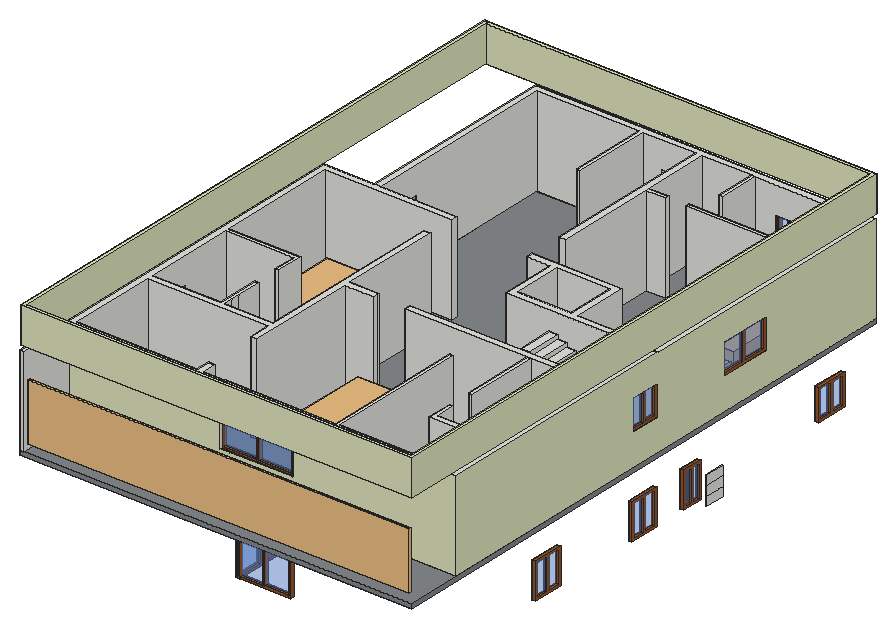
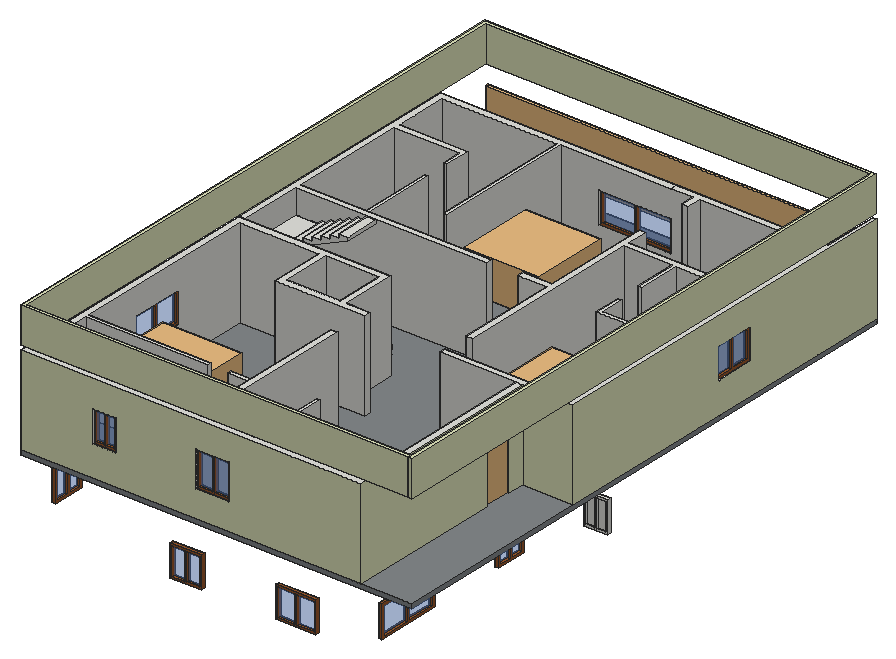
# SketchUp Ruby script. Lengths in inches.
U = 1.inch
M = Sketchup.active_model
def pt(a) = Geom::Point3d.new(a.map { |v| v * U })
def face(e, loops, mat)
  f = e.add_face(loops[0].map { |a| pt(a) })
  loops[1..].each { |l| e.add_face(l.map { |a| pt(a) }).erase! }
  f.material = f.back_material = mat if mat
  f
end
# faces: each face lists its corners as indices into pts; further lists are holes
def faces(e, pts, list, mat = nil) = list.each { |f| face(e, (f[0].is_a?(Array) ? f : [f]).map { |l| l.map { |i| pts[i] } }, mat) }
# xy, xz, yz: faces in a plane at the given z, y or x. An outline is a flat list of corners, or four numbers for a rectangle; further outlines are holes
def ring(l) = l.size == 4 ? [[l[0], l[1]], [l[2], l[1]], [l[2], l[3]], [l[0], l[3]]] : l.each_slice(2).to_a
def flat(e, list, mat, &to3) = list.each { |f| face(e, (f[0].is_a?(Array) ? f : [f]).map { |l| ring(l).map { |u, v| to3.(u, v) } }, mat) }
def xy(e, z, list, mat = nil) = flat(e, list, mat) { |x, y| [x, y, z] }
def xz(e, y, list, mat = nil) = flat(e, list, mat) { |x, z| [x, y, z] }
def yz(e, x, list, mat = nil) = flat(e, list, mat) { |y, z| [x, y, z] }
def lines(e, pts, list) = list.each { |a, b| e.add_line(pt(pts[a]), pt(pts[b])) }
# prism: a flat outline (further loops are holes) pulled along v
def prism(e, loops, v, mat = nil)
  f = face(e, loops, mat); d = Geom::Vector3d.new(v.map { |x| x * U })
  f.pushpull(f.normal.samedirection?(d) ? d.length : -d.length)
end
def box(e, o, s, mat = nil) = prism(e, [[o, [o[0] + s[0], o[1], o[2]], [o[0] + s[0], o[1] + s[1], o[2]], [o[0], o[1] + s[1], o[2]]]], [0, 0, s[2]], mat)
def at(x, y, z, deg = 0) = Geom::Transformation.translation(pt([x, y, z])) * Geom::Transformation.rotation(ORIGIN, Z_AXIS, deg.degrees)
def axes(o, x, y, z) = Geom::Transformation.new([*x, 0, *y, 0, *z, 0, *pt(o).to_a, 1])
def part(name) = M.definitions.add(name)
# library, detail: a bought-in or finely detailed component or shape, given as its bounding box
def library(name, o, s) = part(name).tap { |d| box(d.entities, o, s) }
def detail(e, o, s) = box(e.add_group.entities, o, s)
def put(e, d, t, mat = nil) = e.add_instance(d, t).tap { |i| i.material = mat if mat }
def group(e, t, mat = nil) = e.add_group.tap { |g| g.transformation = t; g.material = mat if mat }.entities
root = M.entities
M.materials.add("0763 AP 7730 GREEN TOMATO").color = [223, 228, 188]
M.materials.add("[Blacktop Old 01]").color = [132, 136, 139]
M.materials.add("[Translucent Glass Blue]").color = [100, 149, 237]
M.materials["[Translucent Glass Blue]"].alpha = 0.5
M.materials.add("[Wood Cherry Original]").color = [152, 86, 42]
c1 = part("Group\#149")
box(c1.entities,[0,-0.08,-0.45],[0.71,26.25,12.58])
c2 = part("Group\#147")
box(c2.entities,[0,-0.08,-0.08],[0.71,26.25,12.21])
c3 = part("Group\#148")
box(c3.entities,[0,-0.08,-0.08],[0.71,26.25,12.21])
c4 = part("Group533\#2")
xy(c4.entities,0,[[-34,-21.5,-1.25,21.5],[1.25,-21.5,34,21.5]])
c5 = part("Group532\#1")
prism(c5.entities,[[[-36.5,-24,0],[-36.5,24,0],[36.5,24,0],[36.5,-24,0]],[[34,21.5,0],[1.25,21.5,0],[1.25,-21.5,0],[34,-21.5,0]],[[-1.25,-21.5,0],[-1.25,21.5,0],[-34,21.5,0],[-34,-21.5,0]]],[0,0,5])
put(c5.entities,c4,at(0,0,2.5),"[Translucent Glass Blue]")
c6 = part("Group549\#2")
xy(c6.entities,0,[[-17.97,-21.5,-1.25,21.5],[1.25,-21.5,17.97,21.5]])
c7 = part("Group548\#1")
prism(c7.entities,[[[-20.47,-24,0],[-20.47,24,0],[20.47,24,0],[20.47,-24,0]],[[-1.25,21.5,0],[-17.97,21.5,0],[-17.97,-21.5,0],[-1.25,-21.5,0]],[[17.97,21.5,0],[1.25,21.5,0],[1.25,-21.5,0],[17.97,-21.5,0]]],[0,0,5])
put(c7.entities,c6,at(0,0,2.5),"[Translucent Glass Blue]")
c8 = part("Group551\#2")
xy(c8.entities,0,[[-18.5,-21.5,-1.25,21.5],[1.25,-21.5,18.5,21.5]])
c9 = part("Group550\#1")
prism(c9.entities,[[[21,24,0],[21,-24,0],[-21,-24,0],[-21,24,0]],[[1.25,-21.5,0],[18.5,-21.5,0],[18.5,21.5,0],[1.25,21.5,0]],[[-1.25,21.5,0],[-18.5,21.5,0],[-18.5,-21.5,0],[-1.25,-21.5,0]]],[0,0,5])
put(c9.entities,c8,at(0,0,2.5),"[Translucent Glass Blue]")
c10 = part("Group547\#2")
xy(c10.entities,0,[[-11.65,-21.5,-1.25,21.5],[1.25,-21.5,11.65,21.5]])
c11 = part("Group546\#1")
prism(c11.entities,[[[-14.15,24,0],[14.15,24,0],[14.15,-24,0],[-14.15,-24,0]],[[1.25,21.5,0],[1.25,-21.5,0],[11.65,-21.5,0],[11.65,21.5,0]],[[-1.25,21.5,0],[-11.65,21.5,0],[-11.65,-21.5,0],[-1.25,-21.5,0]]],[0,0,5])
put(c11.entities,c10,at(0,0,2.5),"[Translucent Glass Blue]")
c12 = part("Group525\#2")
xy(c12.entities,0,[[-24.5,-18.5,-1.25,18.5],[1.25,-18.5,24.5,18.5]])
c13 = part("Group524\#1")
prism(c13.entities,[[[27,-21,0],[-27,-21,0],[-27,21,0],[27,21,0]],[[24.5,-18.5,0],[24.5,18.5,0],[1.25,18.5,0],[1.25,-18.5,0]],[[-1.25,18.5,0],[-24.5,18.5,0],[-24.5,-18.5,0],[-1.25,-18.5,0]]],[0,0,5])
put(c13.entities,c12,at(0,0,2.5),"[Translucent Glass Blue]")
c14 = part("Group527\#2")
xy(c14.entities,0,[[-41.3,-18.5,-1.25,18.5],[1.25,-18.5,41.3,18.5]])
c15 = part("Group526\#1")
prism(c15.entities,[[[-43.8,-21,0],[-43.8,21,0],[43.8,21,0],[43.8,-21,0]],[[-1.25,18.5,0],[-41.3,18.5,0],[-41.3,-18.5,0],[-1.25,-18.5,0]],[[41.3,18.5,0],[1.25,18.5,0],[1.25,-18.5,0],[41.3,-18.5,0]]],[0,0,5])
put(c15.entities,c14,at(0,0,2.5),"[Translucent Glass Blue]")
c16 = part("Group529\#2")
xy(c16.entities,0,[[-13.69,-18.53,-1.25,18.53],[1.25,-18.53,13.69,18.53]])
c17 = part("Group528\#1")
prism(c17.entities,[[[-16.19,21.03,0],[16.19,21.03,0],[16.19,-21.03,0],[-16.19,-21.03,0]],[[1.25,-18.53,0],[13.69,-18.53,0],[13.69,18.53,0],[1.25,18.53,0]],[[-13.69,18.53,0],[-13.69,-18.53,0],[-1.25,-18.53,0],[-1.25,18.53,0]]],[0,0,5])
put(c17.entities,c16,at(0,0,2.5))
c18 = part("Group533\#3")
xy(c18.entities,0,[[-18.39,-18.5,-1.25,18.5],[1.25,-18.5,18.39,18.5]])
c19 = part("Group532\#2")
prism(c19.entities,[[[20.89,-21,0],[-20.89,-21,0],[-20.89,21,0],[20.89,21,0]],[[-1.25,18.5,0],[-18.39,18.5,0],[-18.39,-18.5,0],[-1.25,-18.5,0]],[[18.39,-18.5,0],[18.39,18.5,0],[1.25,18.5,0],[1.25,-18.5,0]]],[0,0,5])
put(c19.entities,c18,at(0,0,2.5),"[Translucent Glass Blue]")
c20 = part("Group545\#2")
xy(c20.entities,0,[[-19.17,-18.5,-1.25,18.5],[1.25,-18.5,19.17,18.5]])
c21 = part("Group544\#1")
prism(c21.entities,[[[21.67,21,0],[21.67,-21,0],[-21.67,-21,0],[-21.67,21,0]],[[-1.25,-18.5,0],[-1.25,18.5,0],[-19.17,18.5,0],[-19.17,-18.5,0]],[[1.25,18.5,0],[1.25,-18.5,0],[19.17,-18.5,0],[19.17,18.5,0]]],[0,0,5])
put(c21.entities,c20,at(0,0,2.5),"[Translucent Glass Blue]")
c22 = part("Group523\#2")
xy(c22.entities,0,[[-18.5,-18.5,-1.25,18.5],[1.25,-18.5,18.5,18.5]])
c23 = part("Group522\#1")
prism(c23.entities,[[[-21,21,0],[21,21,0],[21,-21,0],[-21,-21,0]],[[-1.25,18.5,0],[-18.5,18.5,0],[-18.5,-18.5,0],[-1.25,-18.5,0]],[[18.5,-18.5,0],[18.5,18.5,0],[1.25,18.5,0],[1.25,-18.5,0]]],[0,0,5])
put(c23.entities,c22,at(0,0,2.5),"[Translucent Glass Blue]")
c24 = library("Untitled",[0,0,0],[36,4.39,84])
c25 = library("Table lamp",[7.65,497.27,0],[26.62,26.5,38.96])
c26 = library("bed",[0,0,0],[81.24,78.82,29.53])
c27 = library("Group\#162",[0,0,0],[509.52,3.15,13.86])
c28 = part("Group665\#2")
xy(c28.entities,0,[[-19.73,-21.5,-1.25,21.5],[1.25,-21.5,19.73,21.5]])
c29 = part("Group664\#1")
prism(c29.entities,[[[22.23,-24,0],[-22.23,-24,0],[-22.23,24,0],[22.23,24,0]],[[19.73,21.5,0],[1.25,21.5,0],[1.25,-21.5,0],[19.73,-21.5,0]],[[-1.25,21.5,0],[-19.73,21.5,0],[-19.73,-21.5,0],[-1.25,-21.5,0]]],[0,0,5])
put(c29.entities,c28,at(0,0,2.5),"[Translucent Glass Blue]")
c30 = part("Group663\#2")
xy(c30.entities,0,[[-25.375,-18.5,-1.25,18.5],[1.25,-18.5,25.375,18.5]])
c31 = part("Group662\#1")
prism(c31.entities,[[[-27.875,-21,0],[-27.875,21,0],[27.875,21,0],[27.875,-21,0]],[[-1.25,18.5,0],[-25.375,18.5,0],[-25.375,-18.5,0],[-1.25,-18.5,0]],[[25.375,-18.5,0],[25.375,18.5,0],[1.25,18.5,0],[1.25,-18.5,0]]],[0,0,5])
put(c31.entities,c30,at(0,0,2.5),"[Translucent Glass Blue]")
c32 = part("Group667\#2")
xy(c32.entities,0,[[-12.89,-18.5,-1.25,18.5],[1.25,-18.5,12.89,18.5]])
c33 = part("Group666\#1")
prism(c33.entities,[[[15.39,-21,0],[-15.39,-21,0],[-15.39,21,0],[15.39,21,0]],[[-12.89,18.5,0],[-12.89,-18.5,0],[-1.25,-18.5,0],[-1.25,18.5,0]],[[12.89,-18.5,0],[12.89,18.5,0],[1.25,18.5,0],[1.25,-18.5,0]]],[0,0,5])
put(c33.entities,c32,at(0,0,2.5),"[Translucent Glass Blue]")
c34 = part("Group671\#2")
xy(c34.entities,0,[[-18.5,-18.59,-1.25,18.59],[1.25,-18.59,18.5,18.59]])
c35 = part("Group670\#1")
prism(c35.entities,[[[-21,-21.09,0],[-21,21.09,0],[21,21.09,0],[21,-21.09,0]],[[1.25,18.59,0],[1.25,-18.59,0],[18.5,-18.59,0],[18.5,18.59,0]],[[-1.25,-18.59,0],[-1.25,18.59,0],[-18.5,18.59,0],[-18.5,-18.59,0]]],[0,0,5])
put(c35.entities,c34,at(0,0,2.5),"[Translucent Glass Blue]")
c36 = part("Group673\#2")
xy(c36.entities,0,[[-33.47,-18.5,-1.25,18.5],[1.25,-18.5,33.47,18.5]])
c37 = part("Group672\#1")
prism(c37.entities,[[[35.97,-21,0],[-35.97,-21,0],[-35.97,21,0],[35.97,21,0]],[[-33.47,18.5,0],[-33.47,-18.5,0],[-1.25,-18.5,0],[-1.25,18.5,0]],[[1.25,-18.5,0],[33.47,-18.5,0],[33.47,18.5,0],[1.25,18.5,0]]],[0,0,5])
put(c37.entities,c36,at(0,0,2.5),"[Translucent Glass Blue]")
c38 = part("Group669\#2")
xy(c38.entities,0,[[-45.82,-18.59,-1.25,18.59],[1.25,-18.59,45.82,18.59]])
c39 = part("Group668\#1")
prism(c39.entities,[[[48.32,-21.09,0],[-48.32,-21.09,0],[-48.32,21.09,0],[48.32,21.09,0]],[[45.82,-18.59,0],[45.82,18.59,0],[1.25,18.59,0],[1.25,-18.59,0]],[[-45.82,-18.59,0],[-1.25,-18.59,0],[-1.25,18.59,0],[-45.82,18.59,0]]],[0,0,5])
put(c39.entities,c38,at(0,0,2.5),"[Translucent Glass Blue]")
c40 = part("Group707\#1")
xy(c40.entities,252.1875,[[211.875,172.18,211.875,949.46,216.875,949.46,216.875,177.18,730.875,177.18,730.875,944.46,216.84,944.46,216.84,949.46,735.875,949.46,735.875,172.18]])
xy(c40.entities,300.1875,[[211.875,172.18,735.875,172.18,735.875,949.46,216.84,949.46,216.84,944.46,730.875,944.46,730.875,177.18,216.875,177.18,216.875,949.46,211.875,949.46]])
xz(c40.entities,172.18,[[211.875,252.1875,735.875,300.1875]])
xz(c40.entities,177.18,[[216.875,252.1875,730.875,300.1875]])
xz(c40.entities,944.46,[[216.84,252.1875,730.875,300.1875]])
xz(c40.entities,949.46,[[211.875,252.1875,216.875,300.1875],[216.84,252.1875,735.875,300.1875]])
yz(c40.entities,211.875,[[172.18,252.1875,949.46,300.1875]])
yz(c40.entities,216.84,[[944.46,252.1875,949.46,300.1875]])
yz(c40.entities,216.875,[[177.18,252.1875,949.46,300.1875]])
yz(c40.entities,730.875,[[177.18,252.1875,944.46,300.1875]])
yz(c40.entities,735.875,[[172.18,252.1875,949.46,300.1875]])
put(root,c1,at(344.2,592.79,1.77))
put(root,c2,axes([496.8,582.8125,13.47],[-1,0,0],[0,-1,0],[0,0,-1]))
put(root,c3,axes([496.8,582.8125,25.88],[-1,0,0],[0,-1,0],[0,0,-1]))
put(root,c3,at(344.2,592.79,14.18))
put(root,c1,axes([496.8,582.8125,38.29],[-1,0,0],[0,-1,0],[0,0,-1]))
put(root,c2,at(344.2,592.79,26.59))
put(root,c5,axes([282,83.3,60],[-1,0,0],[0,0,1],[0,1,0]),"[Wood Cherry Original]")
put(root,c7,axes([517,420.83,60],[0,1,0],[0,0,1],[1,0,0]),"[Wood Cherry Original]")
put(root,c9,axes([517,259.53,60],[0,1,0],[0,0,1],[1,0,0]),"[Wood Cherry Original]")
put(root,c5,axes([250.5,119.8,60],[0,-1,0],[0,0,1],[-1,0,0]),"[Wood Cherry Original]")
put(root,c11,axes([517,501.17,60],[0,1,0],[0,0,1],[1,0,0]),"[Wood Cherry Original]")
put(root,c13,axes([156.44,799.3,63],[-1,0,0],[0,0,1],[0,1,0]),"[Wood Cherry Original]")
put(root,c15,axes([75,724.72,63],[0,-1,0],[0,0,1],[-1,0,0]),"[Wood Cherry Original]")
put(root,c17,axes([41.19,442.3,63.03],[-1,0,0],[0,0,1],[0,1,0]))
put(root,c19,axes([75,552.57,63],[0,-1,0],[0,0,1],[-1,0,0]),"[Wood Cherry Original]")
put(root,c21,axes([517,734.16,63],[0,1,0],[0,0,1],[1,0,0]),"[Wood Cherry Original]")
put(root,c23,axes([303.97,799.3,63],[-1,0,0],[0,0,1],[0,1,0]),"[Wood Cherry Original]")
g1 = group(root,at(13,81.3,120),"[Blacktop Old 01]")
box(g1,[-13,-52.28,0],[524,777.28,6])
put(root,c24,at(70.09,596.22,126,-90))
g2 = group(root,at(0,103.3,126))
xy(g2,0,[[0,-74.28,0,136,100,136,100,193.15,105,193.15,105,136,170,136,170,388,179,388,179,254,217.48,254,217.48,245,179,245,179,98.31,170,98.31,170,127,9,127,9,9,29.02,9,29.02,0,5,0,5,-74.28],[29.02,0,29.02,9,170,9,170,28.07,179,28.07,179,9,208.11,9,208.11,0],[208.11,0,208.11,9,356,9,356,198.6,361,198.6,361,9,515,9,515,80,423,80,423,114.95,428,114.95,428,89,515,89,515,245,259.1875,245,259.1875,254,515,254,515,338,524,338,524,0],[0,136,9,191.75],[347,302,359,338],
  [[320,338,320,421,409,421,409,347,515,347,515,520.17,524,520.17,524,338],[329,347,400,412]],[68,492.92,77,560.74],[515,520.17,515,600,350.77,600,350.77,605,515,605,515,694,396.36,694,396.36,703,524,703,524,520.17],[68,560.74,77,592],[213,590,213,694,68,694,68,703,289,703,289,694,218,694,218,590],
  [298,600,324,605]])
xy(g2,36,[[244.54,694,289,703]])
xy(g2,42,[[208.11,0,304.75,9],[0,136,9,191.75],[515,296,524,338],[515,448.23,524,520.17],[396.36,694,427.15,703]])
xy(g2,84,[[0,136,9,191.75],[515,448.23,524,520.17],[68,455.44,77,492.92],[244.54,694,289,703],[396.36,694,427.15,703]])
xy(g2,84.1875,[[208.11,0,304.75,9],[515,296,524,338]])
xy(g2,120,[[0,-74.28,5,-74.28,5,0,208.11,0,208.11,9,179,9,179,28.07,170,28.07,170,9,9,9,9,127,170,127,170,98.31,179,98.31,179,245,217.48,245,217.48,254,179,254,179,388,170,388,170,136,105,136,105,193.15,100,193.15,100,136,9,136,9,258,100,258,100,227.28,105,227.28,105,263,9,263,9,424,179,424,179,433,0,433],[423,146.7,428,245],[[320,338,524,338,524,703,68,703,68,433,77,433,77,694,213,694,213,590,218,590,218,694,289,694,289,465.93,298,465.93,298,694,515,694,515,605,350.77,605,350.77,600,515,600,515,347,409,347,409,421,289,421,289,412,320,412],[329,347,400,412]],[298,600,324,605],[364,639.89,369,694]])
xy(g2,120.1875,[[208.11,0,524,0,524,338,515,338,515,254,259.1875,254,259.1875,245,515,245,515,89,428,89,428,114.95,423,114.95,423,80,515,80,515,9,361,9,361,198.6,356,198.6,356,9,208.11,9]])
xz(g2,-74.28,[[0,0,5,120]])
xz(g2,0,[[[5,0,524,0,524,120.1875,208.11,120.1875,208.11,120,5,120],[208.11,42,304.75,84.1875]]],"0763 AP 7730 GREEN TOMATO")
xz(g2,9,[[9,0,170,120],[[179,0,179,120,208.11,120,208.11,120.1875,356,120.1875,356,0],[208.11,42,304.75,84.1875]],[361,0,515,120.1875]])
xz(g2,28.07,[[170,0,179,120]])
xz(g2,80,[[423,0,515,120.1875]])
xz(g2,89,[[428,0,515,120.1875]])
xz(g2,98.31,[[170,0,179,120]])
xz(g2,114.95,[[423,0,428,120.1875]])
xz(g2,127,[[9,0,170,120]])
xz(g2,136,[[9,0,9,42,0,42,0,84,9,84,9,120,100,120,100,0],[105,0,170,120]])
xz(g2,146.7,[[423,0,428,120]])
xz(g2,191.75,[[0,42,9,84]])
xz(g2,193.15,[[100,0,105,120]])
xz(g2,198.6,[[356,0,361,120.1875]])
xz(g2,227.28,[[100,0,105,120]])
xz(g2,245,[[179,0,217.48,120],[259.1875,0,423,0,423,120,428,120,428,0,515,0,515,120.1875,259.1875,120.1875],[423,0,428,120]])
xz(g2,254,[[179,0,217.48,120],[259.1875,0,515,120.1875]])
xz(g2,258,[[9,0,100,120]])
xz(g2,263,[[9,0,105,120]])
xz(g2,296,[[515,42,524,84.1875]])
xz(g2,338,[[320,0,515,0,515,42,524,42,524,84.1875,515,84.1875,515,120,320,120],[515,120,524,120.1875]])
xz(g2,347,[[329,0,400,120],[409,0,515,120]])
xz(g2,388,[[170,0,179,120]])
xz(g2,412,[[289,0,320,120],[329,0,400,120]])
xz(g2,421,[[289,0,409,120]])
xz(g2,424,[[9,0,179,120]])
xz(g2,433,[[77,0,179,120]])
xz(g2,433,[[0,0,68,120]],"0763 AP 7730 GREEN TOMATO")
xz(g2,448.23,[[515,42,524,84]])
xz(g2,455.44,[[68,0,77,84]],"0763 AP 7730 GREEN TOMATO")
xz(g2,465.93,[[289,0,298,120]])
xz(g2,492.92,[[68,0,77,84]])
xz(g2,520.17,[[515,42,524,84]])
xz(g2,590,[[213,0,218,120]])
xz(g2,600,[[298,0,324,120],[350.77,0,515,120]])
xz(g2,605,[[298,0,324,120],[350.77,0,515,120]])
xz(g2,639.89,[[364,0,369,120]])
xz(g2,694,[[77,0,213,120],[218,0,289,0,289,36,244.54,36,244.54,84,289,84,289,120,218,120],[298,0,364,120],[[369,0,515,120],[396.36,42,427.15,84]]])
xz(g2,703,[[[68,0,524,120],[244.54,36,289,84],[396.36,42,427.15,84]]],"0763 AP 7730 GREEN TOMATO")
yz(g2,0,[[[-74.28,0,433,120],[136,42,191.75,84]]],"0763 AP 7730 GREEN TOMATO")
yz(g2,5,[[-74.28,0,0,120]])
yz(g2,9,[[9,0,127,120],[136,0,258,0,258,120,136,120,136,84,191.75,84,191.75,42,136,42],[263,0,424,120]])
yz(g2,68,[[433,0,433,120,703,120,703,0,492.92,0,492.92,84,455.44,84,455.44,0]],"0763 AP 7730 GREEN TOMATO")
yz(g2,77,[[433,0,455.44,0,455.44,84,492.92,84,492.92,0,694,0,694,120,433,120]])
yz(g2,100,[[136,0,193.15,120],[227.28,0,258,120]])
yz(g2,105,[[136,0,148.1,120],[148.1,0,160,120],[160,0,193.15,120],[227.28,0,263,120]])
yz(g2,170,[[9,0,28.07,120],[98.31,0,127,120],[136,0,388,120]])
yz(g2,179,[[9,0,28.07,120],[98.31,0,245,120],[254,0,388,120],[424,0,433,120]])
yz(g2,208.11,[[0,42,9,84.1875],[0,120,9,120.1875]])
yz(g2,213,[[590,0,694,120]])
yz(g2,217.48,[[245,0,249.55,120],[249.55,0,254,120]])
yz(g2,218,[[590,0,694,120]])
yz(g2,244.54,[[694,36,703,84]])
yz(g2,259.1875,[[245,0,254,120.1875]])
yz(g2,289,[[412,0,421,120],[465.93,0,465.93,120,694,120,694,84,703,84,703,36,694,36,694,0]])
yz(g2,298,[[465.93,0,600,120],[605,0,694,120]])
yz(g2,304.75,[[0,42,9,84.1875]])
yz(g2,320,[[338,0,412,120]])
yz(g2,324,[[600,0,605,120]])
yz(g2,329,[[347,0,412,120]])
yz(g2,350.77,[[600,0,605,120]])
yz(g2,356,[[9,0,198.6,120.1875]])
yz(g2,361,[[9,0,198.6,120.1875]])
yz(g2,364,[[639.89,0,694,120]])
yz(g2,369,[[639.89,0,694,120]])
yz(g2,396.36,[[694,42,703,84]])
yz(g2,400,[[347,0,412,120]])
yz(g2,409,[[347,0,421,120]])
yz(g2,423,[[80,0,114.95,120.1875],[146.7,0,245,120]])
yz(g2,427.15,[[694,42,703,84]])
yz(g2,428,[[89,0,114.95,120.1875],[146.7,0,245,120]])
yz(g2,515,[[9,0,80,120.1875],[89,0,245,120.1875],[254,0,254,120.1875,338,120.1875,338,84.1875,296,84.1875,296,42,338,42,338,0],[[347,0,600,120],[448.23,42,520.17,84]],[605,0,694,120]])
yz(g2,524,[[[0,0,703,0,703,120,338,120,338,120.1875,0,120.1875],[448.23,42,520.17,84],[296,42,338,84.1875]]],"0763 AP 7730 GREEN TOMATO")
# 8992 loose lines left out
put(root,c25,at(477.21,65.07,130.86))
put(root,c26,axes([514.53,682.47,132],[-1.3,0,0],[0,-1.30842,0],[0,0,1.73]))
put(root,c25,axes([479.97,69.46,132],[1.1,0,0],[0,1.21,0],[0,0,0.97387]))
put(root,c25,axes([325.375,-337.59,132],[1.1,0,0],[0,1.21,0],[0,0,0.98416]))
put(root,c26,axes([163.62,469.83,132],[-1.3,0,0],[0,-1.30842,0],[0,0,1.73]))
g3 = group(root,at(347,405.3,132))
prism(g3,[[[168,36,71],[132,36,71],[12,36,1],[12,36,0],[0,36,0],[0,36,7],[12,36,7],[12,36,14],[24,36,14],[24,36,21],[36,36,21],[36,36,28],[48,36,28],[48,36,35],[60,36,35],[60,36,42],[72,36,42],[72,36,49],[84,36,49],[84,36,56],[96,36,56],[96,36,63],[108,36,63],[108,36,70],[120,36,70],[120,36,77],[132,36,77],[132,36,84],[168,36,84]]],[0,-36,0])
put(root,c25,at(322.61,-341.97,140.6))
put(root,c27,axes([16.44,21.45,142.47],[1,0,0],[0,1,0],[0,0,5.56]))
put(root,c26,axes([359.9375,275.43,144.37],[-1.3,0,0],[0,-1.30842,0],[0,0,1.73]))
put(root,c29,axes([266.77,799.3,186],[-1,0,0],[0,0,1],[0,1,0]),"[Wood Cherry Original]")
put(root,c31,axes([7,267.18,189],[0,-1,0],[0,0,1],[-1,0,0]),"[Wood Cherry Original]")
put(root,c33,axes([411.76,799.3,189],[-1,0,0],[0,0,1],[0,1,0]),"[Wood Cherry Original]")
put(root,c35,axes([517,420.3,189.09],[0,1,0],[0,0,1],[1,0,0]),"[Wood Cherry Original]")
put(root,c37,axes([517,587.5,189],[0,1,0],[0,0,1],[1,0,0]),"[Wood Cherry Original]")
put(root,c39,axes([256.43,110.3,189.09],[1,0,0],[0,0,1],[0,-1,0]),"[Wood Cherry Original]")
g4 = group(root,at(407,369.3,209))
prism(g4,[[[0,36,37.1875],[12,36,37.1875],[12,36,31.875],[24,36,31.875],[24,36,26.5625],[36,36,26.5625],[36,36,21.25],[48,36,21.25],[48,36,15.9375],[60,36,15.9375],[60,36,10.625],[72,36,10.625],[72,36,5.3125],[108,36,5.3125],[108,36,0],[72,36,0],[72,36,0.76],[0,36,32.63]]],[0,-48,0])
put(root,c40,at(-211.875,-143.15,0),"0763 AP 7730 GREEN TOMATO")
